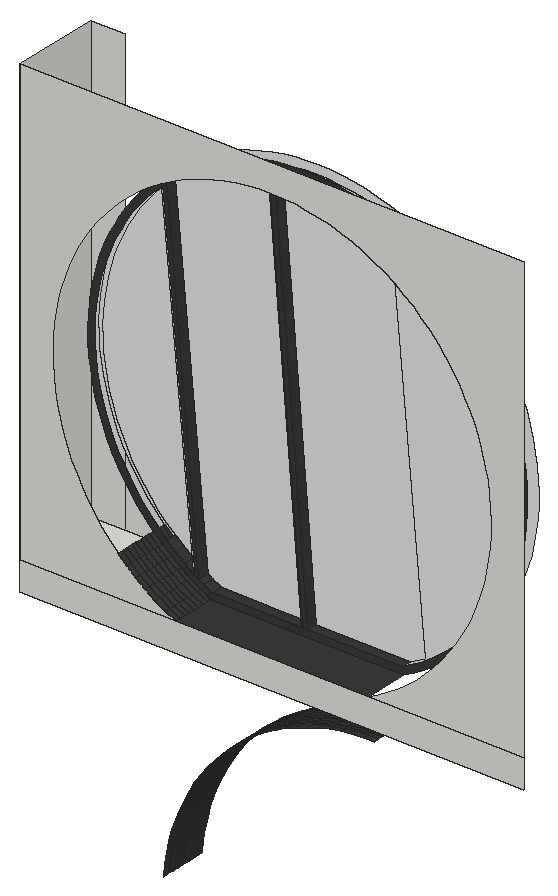
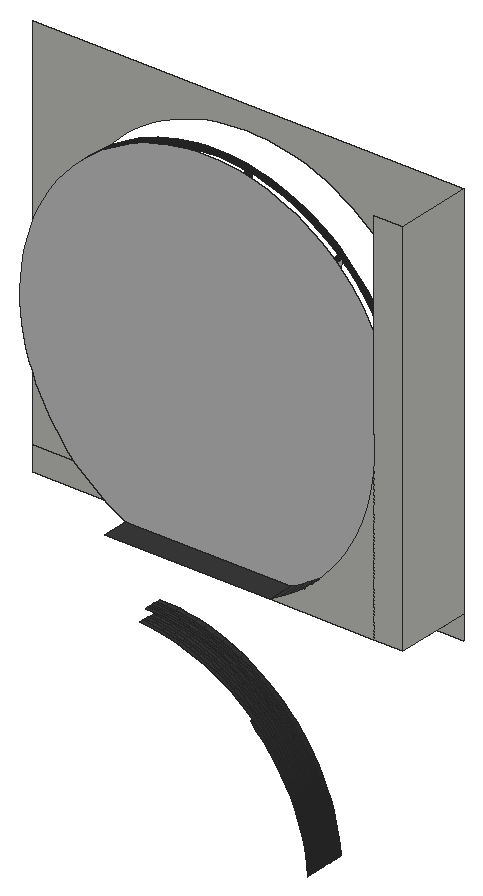
# SketchUp Ruby script. Lengths in inches.
U = 1.inch
M = Sketchup.active_model
def pt(a) = Geom::Point3d.new(a.map { |v| v * U })
def face(e, loops, mat)
  f = e.add_face(loops[0].map { |a| pt(a) })
  loops[1..].each { |l| e.add_face(l.map { |a| pt(a) }).erase! }
  f.material = f.back_material = mat if mat
  f
end
# faces: each face lists its corners as indices into pts; further lists are holes
def faces(e, pts, list, mat = nil) = list.each { |f| face(e, (f[0].is_a?(Array) ? f : [f]).map { |l| l.map { |i| pts[i] } }, mat) }
# xy, xz, yz: faces in a plane at the given z, y or x. An outline is a flat list of corners, or four numbers for a rectangle; further outlines are holes
def ring(l) = l.size == 4 ? [[l[0], l[1]], [l[2], l[1]], [l[2], l[3]], [l[0], l[3]]] : l.each_slice(2).to_a
def flat(e, list, mat, &to3) = list.each { |f| face(e, (f[0].is_a?(Array) ? f : [f]).map { |l| ring(l).map { |u, v| to3.(u, v) } }, mat) }
def xy(e, z, list, mat = nil) = flat(e, list, mat) { |x, y| [x, y, z] }
def xz(e, y, list, mat = nil) = flat(e, list, mat) { |x, z| [x, y, z] }
def yz(e, x, list, mat = nil) = flat(e, list, mat) { |y, z| [x, y, z] }
def lines(e, pts, list) = list.each { |a, b| e.add_line(pt(pts[a]), pt(pts[b])) }
# prism: a flat outline (further loops are holes) pulled along v
def prism(e, loops, v, mat = nil)
  f = face(e, loops, mat); d = Geom::Vector3d.new(v.map { |x| x * U })
  f.pushpull(f.normal.samedirection?(d) ? d.length : -d.length)
end
def box(e, o, s, mat = nil) = prism(e, [[o, [o[0] + s[0], o[1], o[2]], [o[0] + s[0], o[1] + s[1], o[2]], [o[0], o[1] + s[1], o[2]]]], [0, 0, s[2]], mat)
def at(x, y, z, deg = 0) = Geom::Transformation.translation(pt([x, y, z])) * Geom::Transformation.rotation(ORIGIN, Z_AXIS, deg.degrees)
def axes(o, x, y, z) = Geom::Transformation.new([*x, 0, *y, 0, *z, 0, *pt(o).to_a, 1])
def part(name) = M.definitions.add(name)
# library, detail: a bought-in or finely detailed component or shape, given as its bounding box
def library(name, o, s) = part(name).tap { |d| box(d.entities, o, s) }
def detail(e, o, s) = box(e.add_group.entities, o, s)
def put(e, d, t, mat = nil) = e.add_instance(d, t).tap { |i| i.material = mat if mat }
def group(e, t, mat = nil) = e.add_group.tap { |g| g.transformation = t; g.material = mat if mat }.entities
root = M.entities
M.materials.add("[Color M07]").color = [58, 58, 58]
M.materials.add("[Mirror 02]").color = [229, 229, 229]
xy(root,253.6875,[[18.46,0,60.46,1.5],[18.46,1.5,60.46,3],[18.46,3,60.46,4.5],[18.46,4.5,60.46,6],[18.46,6,60.46,7.5],
  [18.46,7.5,60.46,9],[18.46,9,60.46,10.5],[18.46,10.5,60.46,12],[18.46,12,60.46,13.5],[60.46,12,112.46,15.8125],
  [18.46,13.5,60.46,15],[18.46,15,60.46,24]])
xy(root,253.6875,[[60.46,0,112.46,12],[60.46,15.8125,112.46,24]],"[Color M07]")
xy(root,255.52,[[60.91,12,85.02,14.875],[86.46,12,112.01,14.875]],"[Color M07]")
xz(root,0,[[18.46,246,154.46,253.6875],[18.46,253.6875,60.46,253.6875,57.64,255.16,54.89,256.78,52.24,258.55,49.69,260.46,47.25,262.5,44.92,264.68,42.7,266.97,40.62,269.375,38.66,271.89,36.85,274.51,35.18,277.23,33.65,280.02,32.28,282.9,31.07,285.85,30.01,288.85,29.12,291.91,28.39,295.01,27.84,298.15,27.45,301.3125,27.23,304.49,27.18,307.68,27.31,310.86,27.6,314.03,28.06,317.1875,28.7,320.31,29.5,323.39,30.46,326.43,31.59,329.41,32.875,332.33,34.3125,335.17,35.9,337.93,37.64,340.6,39.52,343.17,41.53,345.64,43.67,348,45.94,350.24,48.32,352.36,50.82,354.34,53.42,356.1875,56.11,357.89,58.89,359.45,61.75,360.85,64.68,362.1,67.67,363.19,70.72,364.12,73.8125,364.88,76.94,365.48,80.1,365.91,83.28,366.16,86.46,366.25,89.65,366.16,92.82,365.91,95.98,365.48,99.11,364.88,102.2,364.12,105.25,363.19,108.24,362.1,111.18,360.85,114.04,359.45,116.81,357.89,119.51,356.1875,122.1,354.34,124.6,352.36,126.98,350.24,129.25,348,131.39,345.64,133.4,343.17,135.28,340.6,137.02,337.93,138.61,335.17,140.05,332.33,141.33,329.41,142.46,326.43,143.42,323.39,144.22,320.31,144.86,317.1875,145.32,314.03,145.62,310.86,145.74,307.68,145.69,304.49,145.47,301.3125,145.09,298.15,144.53,295.01,143.8,291.91,142.91,288.85,141.86,285.85,140.64,282.9,139.27,280.02,137.75,277.23,136.07,274.51,134.26,271.89,132.31,269.375,130.22,266.97,128.01,264.68,125.68,262.5,123.23,260.46,120.68,258.55,118.03,256.78,115.29,255.16,112.46,253.6875,154.46,253.6875,154.46,373.6875,18.46,373.6875]])
xz(root,12,[[[60.46,253.6875,112.46,253.6875,115.29,255.16,118.03,256.78,120.68,258.55,123.23,260.46,125.68,262.5,128.01,264.68,130.22,266.97,132.31,269.375,134.26,271.89,136.07,274.51,137.75,277.23,139.27,280.02,140.64,282.9,141.86,285.85,142.91,288.85,143.8,291.91,144.53,295.01,145.09,298.15,145.47,301.3125,145.69,304.49,145.74,307.68,145.62,310.86,145.32,314.03,144.86,317.1875,144.22,320.31,143.42,323.39,142.46,326.43,141.33,329.41,140.05,332.33,138.61,335.17,137.02,337.93,135.28,340.6,133.4,343.17,131.39,345.64,129.25,348,126.98,350.24,124.6,352.36,122.1,354.34,119.51,356.1875,116.81,357.89,114.04,359.45,111.18,360.85,108.24,362.1,105.25,363.19,102.2,364.12,99.11,364.88,95.98,365.48,92.82,365.91,89.65,366.16,86.46,366.25,83.28,366.16,80.1,365.91,76.94,365.48,73.8125,364.88,70.72,364.12,67.67,363.19,64.68,362.1,61.75,360.85,58.89,359.45,56.11,357.89,53.42,356.1875,50.82,354.34,48.32,352.36,45.94,350.24,43.67,348,41.53,345.64,39.52,343.17,37.64,340.6,35.9,337.93,34.3125,335.17,32.875,332.33,31.59,329.41,30.46,326.43,29.5,323.39,28.7,320.31,28.06,317.1875,27.6,314.03,27.31,310.86,27.18,307.68,27.23,304.49,27.45,301.3125,27.84,298.15,28.39,295.01,29.12,291.91,30.01,288.85,31.07,285.85,32.28,282.9,33.65,280.02,35.18,277.23,36.85,274.51,38.66,271.89,40.62,269.375,42.7,266.97,44.92,264.68,47.25,262.5,49.69,260.46,52.24,258.55,54.89,256.78,57.64,255.16],[60.91,255.52,58.53,256.76,57.2,257.55,55.87,258.33,53.3,260.05,50.83,261.9,48.46,263.875,46.2,265.98,44.05,268.2,42.03,270.54,40.14,272.98,38.38,275.51,36.76,278.14,35.28,280.85,33.95,283.64,32.78,286.5,31.75,289.41,30.89,292.375,30.1875,295.38,29.65,298.42,29.27,301.49,29.06,304.57,29.01,307.66,29.13,310.74,29.42,313.82,29.87,316.87,30.48,319.9,31.26,322.89,32.19,325.83,33.28,328.72,34.53,331.54,35.92,334.3,37.47,336.97,39.15,339.5625,40.97,342.06,42.92,344.45,45,346.74,47.19,348.91,48.35,349.93,49.5,350.95,51.92,352.875,54.44,354.67,57.04,356.32,59.74,357.83,62.51,359.19,65.35,360.4,68.25,361.46,71.21,362.36,74.2,363.1,75.72,363.39,77.24,363.67,80.3,364.09,83.375,364.34,86.46,364.42,89.55,364.34,92.625,364.09,95.6875,363.67,98.72,363.1,101.72,362.36,104.67,361.46,107.57,360.4,110.41,359.19,113.18,357.83,115.88,356.32,118.49,354.67,121,352.875,123.42,350.95,125.73,348.91,127.93,346.74,130,344.45,131.95,342.06,133.77,339.5625,135.46,336.97,137,334.3,138.39,331.54,139.64,328.72,140.73,325.83,141.67,322.89,142.44,319.9,143.06,316.87,143.51,313.82,143.79,310.74,143.91,307.66,143.87,304.57,143.65,301.49,143.28,298.42,142.74,295.38,142.03,292.375,141.17,289.41,140.15,286.5,138.97,283.64,137.64,280.85,136.16,278.14,134.54,275.51,132.78,272.98,130.89,270.54,128.87,268.2,126.72,265.98,124.46,263.875,122.09,261.9,119.62,260.05,117.05,258.33,115.72,257.55,114.4,256.76,112.01,255.52]],[85.02,255.52,86.46,255.52,77.24,363.67,75.72,363.39],[57.2,257.55,48.35,349.93,47.19,348.91,55.87,258.33]],"[Color M07]")
xz(root,14.875,[[60.91,255.52,85.02,255.52,75.72,363.39,74.2,363.1,71.21,362.36,68.25,361.46,65.35,360.4,62.51,359.19,59.74,357.83,57.04,356.32,54.44,354.67,51.92,352.875,49.5,350.95,48.35,349.93,57.2,257.55,58.53,256.76],[86.46,255.52,112.01,255.52,114.4,256.76,115.72,257.55,106.12,360.93,104.67,361.46,101.72,362.36,98.72,363.1,95.6875,363.67,92.625,364.09,89.55,364.34,86.46,364.42,83.375,364.34,80.3,364.09,77.24,363.67],[55.87,258.33,47.19,348.91,45,346.74,42.92,344.45,40.97,342.06,39.15,339.5625,37.47,336.97,35.92,334.3,34.53,331.54,33.28,328.72,32.19,325.83,31.26,322.89,30.48,319.9,29.87,316.87,29.42,313.82,29.13,310.74,29.01,307.66,29.06,304.57,29.27,301.49,29.65,298.42,30.1875,295.38,30.89,292.375,31.75,289.41,32.78,286.5,33.95,283.64,35.28,280.85,36.76,278.14,38.38,275.51,40.14,272.98,42.03,270.54,44.05,268.2,46.2,265.98,48.46,263.875,50.83,261.9,53.3,260.05]],"[Mirror 02]")
xz(root,15.8125,[[60.46,253.6875,57.64,255.16,54.89,256.78,52.24,258.55,49.69,260.46,47.25,262.5,44.92,264.68,42.7,266.97,40.62,269.375,38.66,271.89,36.85,274.51,35.18,277.23,33.65,280.02,32.28,282.9,31.07,285.85,30.01,288.85,29.12,291.91,28.39,295.01,27.84,298.15,27.45,301.3125,27.23,304.49,27.18,307.68,27.31,310.86,27.6,314.03,28.06,317.1875,28.7,320.31,29.5,323.39,30.46,326.43,31.59,329.41,32.875,332.33,34.3125,335.17,35.9,337.93,37.64,340.6,39.52,343.17,41.53,345.64,43.67,348,45.94,350.24,48.32,352.36,50.82,354.34,53.42,356.1875,56.11,357.89,58.89,359.45,61.75,360.85,64.68,362.1,67.67,363.19,70.72,364.12,73.8125,364.88,76.94,365.48,80.1,365.91,83.28,366.16,86.46,366.25,89.65,366.16,92.82,365.91,95.98,365.48,99.11,364.88,102.2,364.12,105.25,363.19,108.24,362.1,111.18,360.85,114.04,359.45,116.81,357.89,119.51,356.1875,122.1,354.34,124.6,352.36,126.98,350.24,129.25,348,131.39,345.64,133.4,343.17,135.28,340.6,137.02,337.93,138.61,335.17,140.05,332.33,141.33,329.41,142.46,326.43,143.42,323.39,144.22,320.31,144.86,317.1875,145.32,314.03,145.62,310.86,145.74,307.68,145.69,304.49,145.47,301.3125,145.09,298.15,144.53,295.01,143.8,291.91,142.91,288.85,141.86,285.85,140.64,282.9,139.27,280.02,137.75,277.23,136.07,274.51,134.26,271.89,132.31,269.375,130.22,266.97,128.01,264.68,125.68,262.5,123.23,260.46,120.68,258.55,118.03,256.78,115.29,255.16,112.46,253.6875]],"[Mirror 02]")
xz(root,24,[[18.46,253.6875,18.46,373.6875,27.46,373.6875,27.46,312.54,27.31,310.86,27.18,307.68,27.23,304.49,27.45,301.3125,27.46,301.2,27.46,253.6875],[27.46,253.6875,27.46,301.2,27.84,298.15,28.39,295.01,29.12,291.91,30.01,288.85,31.07,285.85,32.28,282.9,33.65,280.02,35.18,277.23,36.85,274.51,38.66,271.89,40.62,269.375,42.7,266.97,44.92,264.68,47.25,262.5,49.69,260.46,52.24,258.55,54.89,256.78,57.64,255.16,60.46,253.6875]])
yz(root,18.46,[[0,253.6875,24,373.6875]])
p = [[46.5,13.45,181.21],[46.5,14.95,181.21],[46.82,14.95,184.23],[46.82,13.45,184.23],[46.5,15.8,181.21],[46.82,15.8,184.23],
  [46.5,16.65,181.21],[46.82,16.65,184.23],[46.5,17.5,181.21],[46.82,17.5,184.23],[46.5,18.35,181.21],[46.82,18.35,184.23],
  [46.5,19.21,181.21],[46.82,19.21,184.23],[46.5,19.95,181.21],[46.82,19.95,184.23],[46.5,21.02,181.21],[46.82,21.02,184.23],
  [46.5,22.08,181.21],[46.82,22.08,184.23],[46.5,23.14,181.21],[46.82,23.14,184.23],[46.5,24.2,181.21],[46.82,24.2,184.23],
  [46.5,25.27,181.21],[46.82,25.27,184.23],[46.5,26.33,181.21],[46.82,26.33,184.23],[47.3,14.95,187.24],[47.3,13.45,187.24],
  [47.3,15.8,187.24],[47.3,16.65,187.24],[47.3,17.5,187.24],[47.3,18.35,187.24],[47.3,19.21,187.24],[47.3,19.95,187.24],
  [47.3,21.02,187.24],[47.3,22.08,187.24],[47.3,23.14,187.24],[47.3,24.2,187.24],[47.3,25.27,187.24],[47.3,26.33,187.24],
  [47.9375,14.95,190.21],[47.9375,13.45,190.21],[47.9375,15.8,190.21],[47.9375,16.65,190.21],[47.9375,17.5,190.21],[47.9375,18.35,190.21],
  [47.9375,19.21,190.21],[47.9375,19.95,190.21],[47.9375,21.02,190.21],[47.9375,22.08,190.21],[47.9375,23.14,190.21],[47.9375,24.2,190.21],
  [47.9375,25.27,190.21],[47.9375,26.33,190.21],[48.73,14.95,193.15],[48.73,13.45,193.15],[48.73,15.8,193.15],[48.73,16.65,193.15],
  [48.73,17.5,193.15],[48.73,18.35,193.15],[48.73,19.21,193.15],[48.73,19.95,193.15],[48.73,21.02,193.15],[48.73,22.08,193.15],
  [48.73,23.14,193.15],[48.73,24.2,193.15],[48.73,25.27,193.15],[48.73,26.33,193.15],[49.6875,14.95,196.03],[49.6875,13.45,196.03],
  [49.6875,15.8,196.03],[49.6875,16.65,196.03],[49.6875,17.5,196.03],[49.6875,18.35,196.03],[49.6875,19.21,196.03],[49.6875,19.95,196.03],
  [49.6875,21.02,196.03],[49.6875,22.08,196.03],[49.6875,23.14,196.03],[49.6875,24.2,196.03],[49.6875,25.27,196.03],[49.6875,26.33,196.03],
  [50.79,14.95,198.87],[50.79,13.45,198.87],[50.79,15.8,198.87],[50.79,16.65,198.87],[50.79,17.5,198.87],[50.79,18.35,198.87],
  [50.79,19.21,198.87],[50.79,19.95,198.87],[50.79,21.02,198.87],[50.79,22.08,198.87],[50.79,23.14,198.87],[50.79,24.2,198.87],
  [50.79,25.27,198.87],[50.79,26.33,198.87],[52.05,14.95,201.64],[52.05,13.45,201.64],[52.05,15.8,201.64],[52.05,16.65,201.64],
  [52.05,17.5,201.64],[52.05,18.35,201.64],[52.05,19.21,201.64],[52.05,19.95,201.64],[52.05,21.02,201.64],[52.05,22.08,201.64],
  [52.05,23.14,201.64],[52.05,24.2,201.64],[52.05,25.27,201.64],[52.05,26.33,201.64],[53.45,14.95,204.34],[53.45,13.45,204.34],
  [53.45,15.8,204.34],[53.45,16.65,204.34],[53.45,17.5,204.34],[53.45,18.35,204.34],[53.45,19.21,204.34],[53.45,19.95,204.34],
  [53.45,21.02,204.34],[53.45,22.08,204.34],[53.45,23.14,204.34],[53.45,24.2,204.34],[53.45,25.27,204.34],[53.45,26.33,204.34],
  [54.99,14.95,206.96],[54.99,13.45,206.96],[54.99,15.8,206.96],[54.99,16.65,206.96],[54.99,17.5,206.96],[54.99,18.35,206.96],
  [54.99,19.21,206.96],[54.99,19.95,206.96],[54.99,21.02,206.96],[54.99,22.08,206.96],[54.99,23.14,206.96],[54.99,24.2,206.96],
  [54.99,25.27,206.96],[54.99,26.33,206.96],[56.67,14.95,209.5],[56.67,13.45,209.5],[56.67,15.8,209.5],[56.67,16.65,209.5],
  [56.67,17.5,209.5],[56.67,18.35,209.5],[56.67,19.21,209.5],[56.67,19.95,209.5],[56.67,21.02,209.5],[56.67,22.08,209.5],
  [56.67,23.14,209.5],[56.67,24.2,209.5],[56.67,25.27,209.5],[56.67,26.33,209.5],[58.48,14.95,211.94],[58.48,13.45,211.94],
  [58.48,15.8,211.94],[58.48,16.65,211.94],[58.48,17.5,211.94],[58.48,18.35,211.94],[58.48,19.21,211.94],[58.48,19.95,211.94],
  [58.48,21.02,211.94],[58.48,22.08,211.94],[58.48,23.14,211.94],[58.48,24.2,211.94],[58.48,25.27,211.94],[58.48,26.33,211.94],
  [60.42,14.95,214.29],[60.42,13.45,214.29],[60.42,15.8,214.29],[60.42,16.65,214.29],[60.42,17.5,214.29],[60.42,18.35,214.29],
  [60.42,19.21,214.29],[60.42,19.95,214.29],[60.42,21.02,214.29],[60.42,22.08,214.29],[60.42,23.14,214.29],[60.42,24.2,214.29],
  [60.42,25.27,214.29],[60.42,26.33,214.29],[62.48,14.95,216.52],[62.48,13.45,216.52],[62.48,15.8,216.52],[62.48,16.65,216.52],
  [62.48,17.5,216.52],[62.48,18.35,216.52],[62.48,19.21,216.52],[62.48,19.95,216.52],[62.48,21.02,216.52],[62.48,22.08,216.52],
  [62.48,23.14,216.52],[62.48,24.2,216.52],[62.48,25.27,216.52],[62.48,26.33,216.52],[64.66,14.95,218.65],[64.66,13.45,218.65],
  [64.66,15.8,218.65],[64.66,16.65,218.65],[64.66,17.5,218.65],[64.66,18.35,218.65],[64.66,19.21,218.65],[64.66,19.95,218.65],
  [64.66,21.02,218.65],[64.66,22.08,218.65],[64.66,23.14,218.65],[64.66,24.2,218.65],[64.66,25.27,218.65],[64.66,26.33,218.65],
  [66.95,14.95,220.65],[66.95,13.45,220.65],[66.95,15.8,220.65],[66.95,16.65,220.65],[66.95,17.5,220.65],[66.95,18.35,220.65],
  [66.95,19.21,220.65],[66.95,19.95,220.65],[66.95,21.02,220.65],[66.95,22.08,220.65],[66.95,23.14,220.65],[66.95,24.2,220.65],
  [66.95,25.27,220.65],[69.34,14.95,222.53],[69.34,13.45,222.53],[69.34,15.8,222.53],[69.34,16.65,222.53],[69.34,17.5,222.53],
  [69.34,18.35,222.53],[69.34,19.21,222.53],[69.34,19.95,222.53],[69.34,21.02,222.53],[69.34,22.08,222.53],[69.34,23.14,222.53],
  [69.34,24.2,222.53],[69.34,25.27,222.53],[71.83,14.95,224.28],[71.83,13.45,224.28],[71.83,15.8,224.28],[71.83,16.65,224.28],
  [71.83,17.5,224.28],[71.83,18.35,224.28],[71.83,19.21,224.28],[71.83,19.95,224.28],[71.83,21.02,224.28],[71.83,22.08,224.28],
  [71.83,23.14,224.28],[71.83,24.2,224.28],[71.83,25.27,224.28],[74.41,14.95,225.9],[74.41,13.45,225.9],[74.41,15.8,225.9],
  [74.41,16.65,225.9],[74.41,17.5,225.9],[74.41,18.35,225.9],[74.41,19.21,225.9],[74.41,19.95,225.9],[74.41,21.02,225.9],
  [74.41,22.08,225.9],[74.41,23.14,225.9],[74.41,24.2,225.9],[74.41,25.27,225.9],[77.07,14.95,227.37],[77.07,13.45,227.37],
  [77.07,15.8,227.37],[77.07,16.65,227.37],[77.07,17.5,227.37],[77.07,18.35,227.37],[77.07,19.21,227.37],[77.07,19.95,227.37],
  [77.07,21.02,227.37],[77.07,22.08,227.37],[77.07,23.14,227.37],[77.07,24.2,227.37],[77.07,25.27,227.37],[79.81,14.95,228.7],
  [79.81,13.45,228.7],[79.81,15.8,228.7],[79.81,16.65,228.7],[79.81,17.5,228.7],[79.81,18.35,228.7],[79.81,19.21,228.7],
  [79.81,19.95,228.7],[79.81,21.02,228.7],[79.81,22.08,228.7],[79.81,23.14,228.7],[79.81,24.2,228.7],[79.81,25.27,228.7],
  [82.61,14.95,229.89],[82.61,13.45,229.89],[82.61,15.8,229.89],[82.61,16.65,229.89],[82.61,17.5,229.89],[82.61,18.35,229.89],
  [82.61,19.21,229.89],[82.61,19.95,229.89],[82.61,21.02,229.89],[82.61,22.08,229.89],[82.61,23.14,229.89],[82.61,24.2,229.89],
  [82.61,25.27,229.89],[85.47,14.95,230.92],[85.47,13.45,230.92],[85.47,15.8,230.92],[85.47,16.65,230.92],[85.47,17.5,230.92],
  [85.47,18.35,230.92],[85.47,19.21,230.92],[85.47,19.95,230.92],[85.47,21.02,230.92],[85.47,22.08,230.92],[85.47,23.14,230.92],
  [85.47,24.2,230.92],[85.47,25.27,230.92],[88.38,14.95,231.8],[88.38,13.45,231.8],[88.38,15.8,231.8],[88.38,16.65,231.8],
  [88.38,17.5,231.8],[88.38,18.35,231.8],[88.38,19.21,231.8],[88.38,19.95,231.8],[88.38,21.02,231.8],[88.38,22.08,231.8],
  [88.38,23.14,231.8],[88.38,24.2,231.8],[88.38,25.27,231.8],[91.34,14.95,232.52],[91.34,13.45,232.52],[91.34,15.8,232.52],
  [91.34,16.65,232.52],[91.34,17.5,232.52],[91.34,18.35,232.52],[91.34,19.21,232.52],[91.34,19.95,232.52],[91.34,21.02,232.52],
  [91.34,22.08,232.52],[91.34,23.14,232.52],[91.34,24.2,232.52],[91.34,25.27,232.52],[94.33,14.95,233.08],[94.33,13.45,233.08],
  [94.33,15.8,233.08],[94.33,16.65,233.08],[94.33,17.5,233.08],[94.33,18.35,233.08],[94.33,19.21,233.08],[94.33,19.95,233.08],
  [94.33,21.02,233.08],[94.33,22.08,233.08],[94.33,23.14,233.08],[94.33,24.2,233.08],[94.33,25.27,233.08],[97.34,14.95,233.49],
  [97.34,13.45,233.49],[97.34,15.8,233.49],[97.34,16.65,233.49],[97.34,17.5,233.49],[97.34,18.35,233.49],[97.34,19.21,233.49],
  [97.34,19.95,233.49],[97.34,21.02,233.49],[97.34,22.08,233.49],[97.34,23.14,233.49],[97.34,24.2,233.49],[97.34,25.27,233.49],
  [100.375,14.95,233.73],[100.375,13.45,233.73],[100.375,15.8,233.73],[100.375,16.65,233.73],[100.375,17.5,233.73],[100.375,18.35,233.73],
  [100.375,19.21,233.73],[100.375,19.95,233.73],[100.375,21.02,233.73],[100.375,22.08,233.73],[100.375,23.14,233.73],[100.375,24.2,233.73],
  [100.375,25.27,233.73],[103.41,14.95,233.8125],[103.41,13.45,233.8125],[103.41,15.8,233.8125],[103.41,16.65,233.8125],[103.41,17.5,233.8125],
  [103.41,18.35,233.8125],[103.41,19.21,233.8125],[60.46,0,253.6875],[60.46,1.5,253.6875],[57.64,1.5,255.16],[57.64,0,255.16],
  [60.46,3,253.6875],[57.64,3,255.16],[60.46,4.5,253.6875],[57.64,4.5,255.16],[60.46,6,253.6875],[57.64,6,255.16],
  [60.46,7.5,253.6875],[57.64,7.5,255.16],[60.46,9,253.6875],[57.64,9,255.16],[60.46,10.5,253.6875],[57.64,10.5,255.16],
  [60.46,12,253.6875],[57.64,12,255.16],[60.46,13.5,253.6875],[57.64,13.5,255.16],[60.46,15,253.6875],[57.64,15,255.16],
  [60.46,15.8125,253.6875],[57.64,15.8125,255.16],[57.64,24,255.16],[60.46,24,253.6875],[54.89,1.5,256.78],[54.89,0,256.78],
  [54.89,3,256.78],[54.89,4.5,256.78],[54.89,6,256.78],[54.89,7.5,256.78],[54.89,9,256.78],[54.89,10.5,256.78],
  [54.89,12,256.78],[54.89,13.5,256.78],[54.89,15,256.78],[54.89,15.8125,256.78],[54.89,24,256.78],[60.91,14.875,255.52],
  [58.53,14.875,256.76],[58.53,12,256.76],[60.91,12,255.52],[75.72,14.875,363.39],[85.02,14.875,255.52],[85.02,12,255.52],
  [75.72,12,363.39],[86.46,14.875,255.52],[77.24,14.875,363.67],[77.24,12,363.67],[86.46,12,255.52],[52.24,1.5,258.55],
  [52.24,0,258.55],[52.24,3,258.55],[52.24,4.5,258.55],[52.24,6,258.55],[52.24,7.5,258.55],[52.24,9,258.55],
  [52.24,10.5,258.55],[52.24,12,258.55],[52.24,13.5,258.55],[57.2,14.875,257.55],[57.2,12,257.55],[52.24,15,258.55],
  [52.24,15.8125,258.55],[52.24,24,258.55],[48.35,14.875,349.93],[48.35,12,349.93],[47.19,14.875,348.91],[55.87,14.875,258.33],
  [55.87,12,258.33],[47.19,12,348.91],[53.3,14.875,260.05],[53.3,12,260.05],[49.69,1.5,260.46],[49.69,0,260.46],
  [49.69,3,260.46],[49.69,4.5,260.46],[49.69,6,260.46],[49.69,7.5,260.46],[49.69,9,260.46],[49.69,10.5,260.46],
  [49.69,12,260.46],[49.69,13.5,260.46],[49.69,15,260.46],[49.69,15.8125,260.46],[49.69,24,260.46],[50.83,14.875,261.9],
  [50.83,12,261.9],[47.25,1.5,262.5],[47.25,0,262.5],[47.25,3,262.5],[47.25,4.5,262.5],[47.25,6,262.5],
  [47.25,7.5,262.5],[47.25,9,262.5],[47.25,10.5,262.5],[47.25,12,262.5],[47.25,13.5,262.5],[47.25,15,262.5],
  [47.25,15.8125,262.5],[47.25,24,262.5],[48.46,14.875,263.875],[48.46,12,263.875],[44.92,1.5,264.68],[44.92,0,264.68],
  [44.92,3,264.68],[44.92,4.5,264.68],[44.92,6,264.68],[44.92,7.5,264.68],[44.92,9,264.68],[44.92,10.5,264.68],
  [44.92,12,264.68],[44.92,13.5,264.68],[44.92,15,264.68],[44.92,15.8125,264.68],[44.92,24,264.68],[41.2,13.45,246],
  [41.2,13.45,252]]
faces(root,p,[[0,1,2,3],[1,4,5,2],[4,6,7,5],[6,8,9,7],[8,10,11,9],[10,12,13,11],[12,14,15,13],[14,16,17,15],
  [16,18,19,17],[18,20,21,19],[20,22,23,21],[22,24,25,23],[24,26,27,25],[3,2,28,29],[2,5,30,28],[5,7,31,30],
  [7,9,32,31],[9,11,33,32],[11,13,34,33],[13,15,35,34],[15,17,36,35],[17,19,37,36],[19,21,38,37],[21,23,39,38],
  [23,25,40,39],[25,27,41,40],[29,28,42,43],[28,30,44,42],[30,31,45,44],[31,32,46,45],[32,33,47,46],[33,34,48,47],
  [34,35,49,48],[35,36,50,49],[36,37,51,50],[37,38,52,51],[38,39,53,52],[39,40,54,53],[40,41,55,54],[43,42,56,57],
  [42,44,58,56],[44,45,59,58],[45,46,60,59],[46,47,61,60],[47,48,62,61],[48,49,63,62],[49,50,64,63],[50,51,65,64],
  [51,52,66,65],[52,53,67,66],[53,54,68,67],[54,55,69,68],[57,56,70,71],[56,58,72,70],[58,59,73,72],[59,60,74,73],
  [60,61,75,74],[61,62,76,75],[62,63,77,76],[63,64,78,77],[64,65,79,78],[65,66,80,79],[66,67,81,80],[67,68,82,81],
  [68,69,83,82],[71,70,84,85],[70,72,86,84],[72,73,87,86],[73,74,88,87],[74,75,89,88],[75,76,90,89],[76,77,91,90],
  [77,78,92,91],[78,79,93,92],[79,80,94,93],[80,81,95,94],[81,82,96,95],[82,83,97,96],[85,84,98,99],[84,86,100,98],
  [86,87,101,100],[87,88,102,101],[88,89,103,102],[89,90,104,103],[90,91,105,104],[91,92,106,105],[92,93,107,106],[93,94,108,107],
  [94,95,109,108],[95,96,110,109],[96,97,111,110],[99,98,112,113],[98,100,114,112],[100,101,115,114],[101,102,116,115],[102,103,117,116],
  [103,104,118,117],[104,105,119,118],[105,106,120,119],[106,107,121,120],[107,108,122,121],[108,109,123,122],[109,110,124,123],[110,111,125,124],
  [113,112,126,127],[112,114,128,126],[114,115,129,128],[115,116,130,129],[116,117,131,130],[117,118,132,131],[118,119,133,132],[119,120,134,133],
  [120,121,135,134],[121,122,136,135],[122,123,137,136],[123,124,138,137],[124,125,139,138],[127,126,140,141],[126,128,142,140],[128,129,143,142],
  [129,130,144,143],[130,131,145,144],[131,132,146,145],[132,133,147,146],[133,134,148,147],[134,135,149,148],[135,136,150,149],[136,137,151,150],
  [137,138,152,151],[138,139,153,152],[141,140,154,155],[140,142,156,154],[142,143,157,156],[143,144,158,157],[144,145,159,158],[145,146,160,159],
  [146,147,161,160],[147,148,162,161],[148,149,163,162],[149,150,164,163],[150,151,165,164],[151,152,166,165],[152,153,167,166],[155,154,168,169],
  [154,156,170,168],[156,157,171,170],[157,158,172,171],[158,159,173,172],[159,160,174,173],[160,161,175,174],[161,162,176,175],[162,163,177,176],
  [163,164,178,177],[164,165,179,178],[165,166,180,179],[166,167,181,180],[169,168,182,183],[168,170,184,182],[170,171,185,184],[171,172,186,185],
  [172,173,187,186],[173,174,188,187],[174,175,189,188],[175,176,190,189],[176,177,191,190],[177,178,192,191],[178,179,193,192],[179,180,194,193],
  [180,181,195,194],[183,182,196,197],[182,184,198,196],[184,185,199,198],[185,186,200,199],[186,187,201,200],[187,188,202,201],[188,189,203,202],
  [189,190,204,203],[190,191,205,204],[191,192,206,205],[192,193,207,206],[193,194,208,207],[194,195,209,208],[197,196,210,211],[196,198,212,210],
  [198,199,213,212],[199,200,214,213],[200,201,215,214],[201,202,216,215],[202,203,217,216],[203,204,218,217],[204,205,219,218],[205,206,220,219],
  [206,207,221,220],[207,208,222,221],[211,210,223,224],[210,212,225,223],[212,213,226,225],[213,214,227,226],[214,215,228,227],[215,216,229,228],
  [216,217,230,229],[217,218,231,230],[218,219,232,231],[219,220,233,232],[220,221,234,233],[221,222,235,234],[224,223,236,237],[223,225,238,236],
  [225,226,239,238],[226,227,240,239],[227,228,241,240],[228,229,242,241],[229,230,243,242],[230,231,244,243],[231,232,245,244],[232,233,246,245],
  [233,234,247,246],[234,235,248,247],[237,236,249,250],[236,238,251,249],[238,239,252,251],[239,240,253,252],[240,241,254,253],[241,242,255,254],
  [242,243,256,255],[243,244,257,256],[244,245,258,257],[245,246,259,258],[246,247,260,259],[247,248,261,260],[250,249,262,263],[249,251,264,262],
  [251,252,265,264],[252,253,266,265],[253,254,267,266],[254,255,268,267],[255,256,269,268],[256,257,270,269],[257,258,271,270],[258,259,272,271],
  [259,260,273,272],[260,261,274,273],[263,262,275,276],[262,264,277,275],[264,265,278,277],[265,266,279,278],[266,267,280,279],[267,268,281,280],
  [268,269,282,281],[269,270,283,282],[270,271,284,283],[271,272,285,284],[272,273,286,285],[273,274,287,286],[276,275,288,289],[275,277,290,288],
  [277,278,291,290],[278,279,292,291],[279,280,293,292],[280,281,294,293],[281,282,295,294],[282,283,296,295],[283,284,297,296],[284,285,298,297],
  [285,286,299,298],[286,287,300,299],[289,288,301,302],[288,290,303,301],[290,291,304,303],[291,292,305,304],[292,293,306,305],[293,294,307,306],
  [294,295,308,307],[295,296,309,308],[296,297,310,309],[297,298,311,310],[298,299,312,311],[299,300,313,312],[302,301,314,315],[301,303,316,314],
  [303,304,317,316],[304,305,318,317],[305,306,319,318],[306,307,320,319],[307,308,321,320],[308,309,322,321],[309,310,323,322],[310,311,324,323],
  [311,312,325,324],[312,313,326,325],[315,314,327,328],[314,316,329,327],[316,317,330,329],[317,318,331,330],[318,319,332,331],[319,320,333,332],
  [320,321,334,333],[321,322,335,334],[322,323,336,335],[323,324,337,336],[324,325,338,337],[325,326,339,338],[328,327,340,341],[327,329,342,340],
  [329,330,343,342],[330,331,344,343],[331,332,345,344],[332,333,346,345],[333,334,347,346],[334,335,348,347],[335,336,349,348],[336,337,350,349],
  [337,338,351,350],[338,339,352,351],[341,340,353,354],[340,342,355,353],[342,343,356,355],[343,344,357,356],[344,345,358,357],[345,346,359,358],
  [346,347,360,359],[347,348,361,360],[348,349,362,361],[349,350,363,362],[350,351,364,363],[351,352,365,364],[354,353,366,367],[353,355,368,366],
  [355,356,369,368],[356,357,370,369],[357,358,371,370],[358,359,372,371],[359,360,373,372],[360,361,374,373],[361,362,375,374],[362,363,376,375],
  [363,364,377,376],[364,365,378,377],[367,366,379,380],[366,368,381,379],[368,369,382,381],[369,370,383,382],[370,371,384,383],[371,372,385,384],
  [386,387,388,389],[387,390,391,388],[390,392,393,391],[392,394,395,393],[394,396,397,395],[396,398,399,397],[398,400,401,399],[400,402,403,401],
  [404,402,403,405],[406,404,405,407],[408,409,407,406],[410,409,408,411],[389,388,412,413],[388,391,414,412],[391,393,415,414],[393,395,416,415],
  [395,397,417,416],[397,399,418,417],[399,401,419,418],[401,403,420,419],[405,403,420,421],[407,405,421,422],[409,423,422,407],[424,423,409,410],
  [425,426,427,428],[429,430,431,432],[433,434,435,436],[413,412,437,438],[412,414,439,437],[414,415,440,439],[415,416,441,440],[416,417,442,441],
  [417,418,443,442],[418,419,444,443],[419,420,445,444],[421,420,445,446],[426,447,448,427],[422,421,446,449],[423,450,449,422],[451,450,423,424],
  [447,452,453,448],[455,458,459,456],[438,437,460,461],[437,439,462,460],[439,440,463,462],[440,441,464,463],[441,442,465,464],[442,443,466,465],
  [443,444,467,466],[444,445,468,467],[446,445,468,469],[449,446,469,470],[450,471,470,449],[472,471,450,451],[458,473,474,459],[461,460,475,476],
  [460,462,477,475],[462,463,478,477],[463,464,479,478],[464,465,480,479],[465,466,481,480],[466,467,482,481],[467,468,483,482],[469,468,483,484],
  [470,469,484,485],[471,486,485,470],[487,486,471,472],[473,488,489,474],[476,475,490,491],[475,477,492,490],[477,478,493,492],[478,479,494,493],
  [479,480,495,494],[480,481,496,495],[481,482,497,496],[482,483,498,497],[484,483,498,499],[485,484,499,500],[486,501,500,485],[502,501,486,487]],"[Color M07]")
faces(root,p,[[454,455,456,457]])
lines(root,p,[[503,504]])
